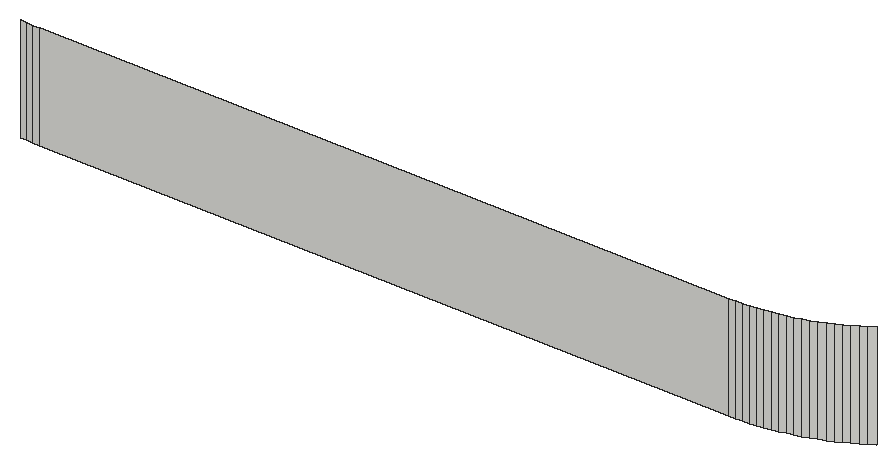
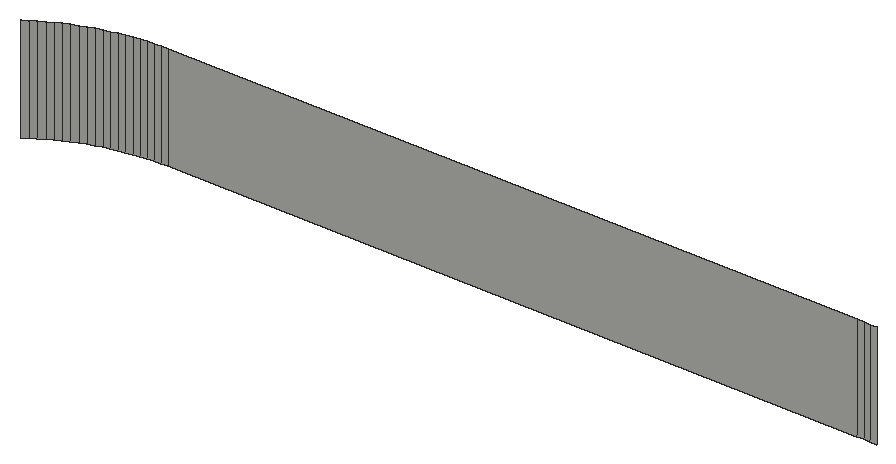
# SketchUp Ruby script. Lengths in inches.
U = 1.inch
M = Sketchup.active_model
def pt(a) = Geom::Point3d.new(a.map { |v| v * U })
def face(e, loops, mat)
  f = e.add_face(loops[0].map { |a| pt(a) })
  loops[1..].each { |l| e.add_face(l.map { |a| pt(a) }).erase! }
  f.material = f.back_material = mat if mat
  f
end
# faces: each face lists its corners as indices into pts; further lists are holes
def faces(e, pts, list, mat = nil) = list.each { |f| face(e, (f[0].is_a?(Array) ? f : [f]).map { |l| l.map { |i| pts[i] } }, mat) }
# xy, xz, yz: faces in a plane at the given z, y or x. An outline is a flat list of corners, or four numbers for a rectangle; further outlines are holes
def ring(l) = l.size == 4 ? [[l[0], l[1]], [l[2], l[1]], [l[2], l[3]], [l[0], l[3]]] : l.each_slice(2).to_a
def flat(e, list, mat, &to3) = list.each { |f| face(e, (f[0].is_a?(Array) ? f : [f]).map { |l| ring(l).map { |u, v| to3.(u, v) } }, mat) }
def xy(e, z, list, mat = nil) = flat(e, list, mat) { |x, y| [x, y, z] }
def xz(e, y, list, mat = nil) = flat(e, list, mat) { |x, z| [x, y, z] }
def yz(e, x, list, mat = nil) = flat(e, list, mat) { |y, z| [x, y, z] }
def lines(e, pts, list) = list.each { |a, b| e.add_line(pt(pts[a]), pt(pts[b])) }
# prism: a flat outline (further loops are holes) pulled along v
def prism(e, loops, v, mat = nil)
  f = face(e, loops, mat); d = Geom::Vector3d.new(v.map { |x| x * U })
  f.pushpull(f.normal.samedirection?(d) ? d.length : -d.length)
end
def box(e, o, s, mat = nil) = prism(e, [[o, [o[0] + s[0], o[1], o[2]], [o[0] + s[0], o[1] + s[1], o[2]], [o[0], o[1] + s[1], o[2]]]], [0, 0, s[2]], mat)
def at(x, y, z, deg = 0) = Geom::Transformation.translation(pt([x, y, z])) * Geom::Transformation.rotation(ORIGIN, Z_AXIS, deg.degrees)
def axes(o, x, y, z) = Geom::Transformation.new([*x, 0, *y, 0, *z, 0, *pt(o).to_a, 1])
def part(name) = M.definitions.add(name)
# library, detail: a bought-in or finely detailed component or shape, given as its bounding box
def library(name, o, s) = part(name).tap { |d| box(d.entities, o, s) }
def detail(e, o, s) = box(e.add_group.entities, o, s)
def put(e, d, t, mat = nil) = e.add_instance(d, t).tap { |i| i.material = mat if mat }
def group(e, t, mat = nil) = e.add_group.tap { |g| g.transformation = t; g.material = mat if mat }.entities
root = M.entities
xz(root,228,[[82,348,141,357]])
p = [[80.31,228.08,357],[80.87,228.04,357],[80.87,228.04,348],[80.31,228.08,348],[81.43,228.01,357],[81.43,228.01,348],
  [82,228,357],[82,228,348],[141,228,357],[141.57,228.01,357],[141.57,228.01,348],[141,228,348],
  [142.13,228.04,357],[142.13,228.04,348],[142.69,228.08,357],[142.69,228.08,348],[143.26,228.14,357],[143.26,228.14,348],
  [143.82,228.22,357],[143.82,228.22,348],[144.37,228.32,357],[144.37,228.32,348],[144.93,228.43,357],[144.93,228.43,348],
  [145.48,228.57,357],[145.48,228.57,348],[146.02,228.71,357],[146.02,228.71,348],[146.5625,228.88,357],[146.5625,228.88,348],
  [147.1,229.0625,357],[147.1,229.0625,348],[147.625,229.26,357],[147.625,229.26,348],[148.15,229.48,357],[148.15,229.48,348],
  [148.66,229.71,357],[148.66,229.71,348],[149.17,229.96,357],[149.17,229.96,348],[149.67,230.23,357],[149.67,230.23,348],
  [150.16,230.51,357],[150.16,230.51,348],[150.64,230.8,357],[150.64,230.8,348],[151.12,231.11,357],[151.12,231.11,348]]
faces(root,p,[[0,1,2,3],[1,4,5,2],[4,6,7,5],[8,9,10,11],[9,12,13,10],[12,14,15,13],[14,16,17,15],[16,18,19,17],
  [18,20,21,19],[20,22,23,21],[22,24,25,23],[24,26,27,25],[26,28,29,27],[28,30,31,29],[30,32,33,31],[32,34,35,33],
  [34,36,37,35],[36,38,39,37],[38,40,41,39],[40,42,43,41],[42,44,45,43],[44,46,47,45]])
